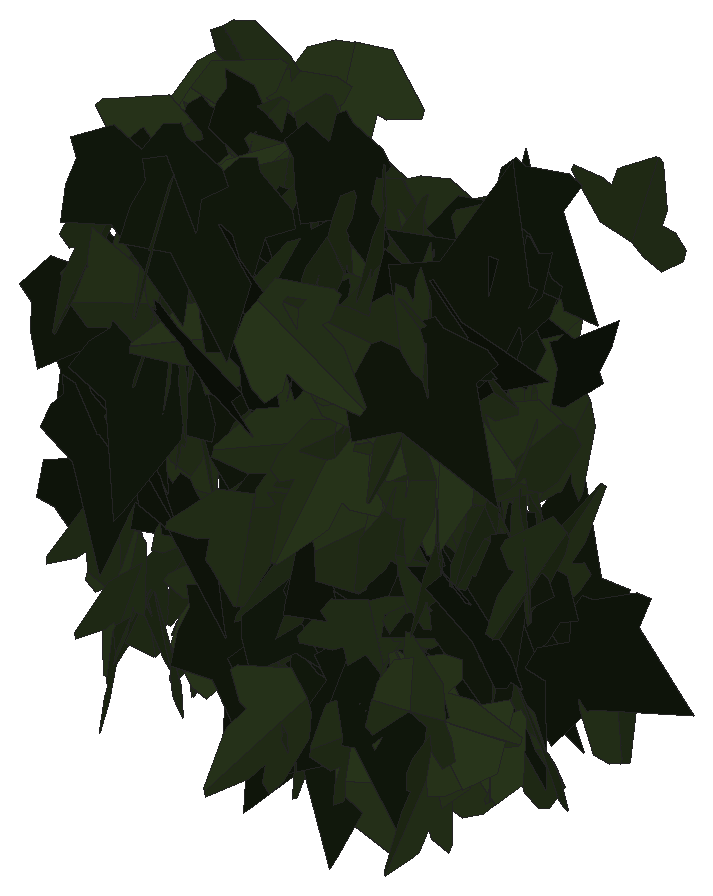
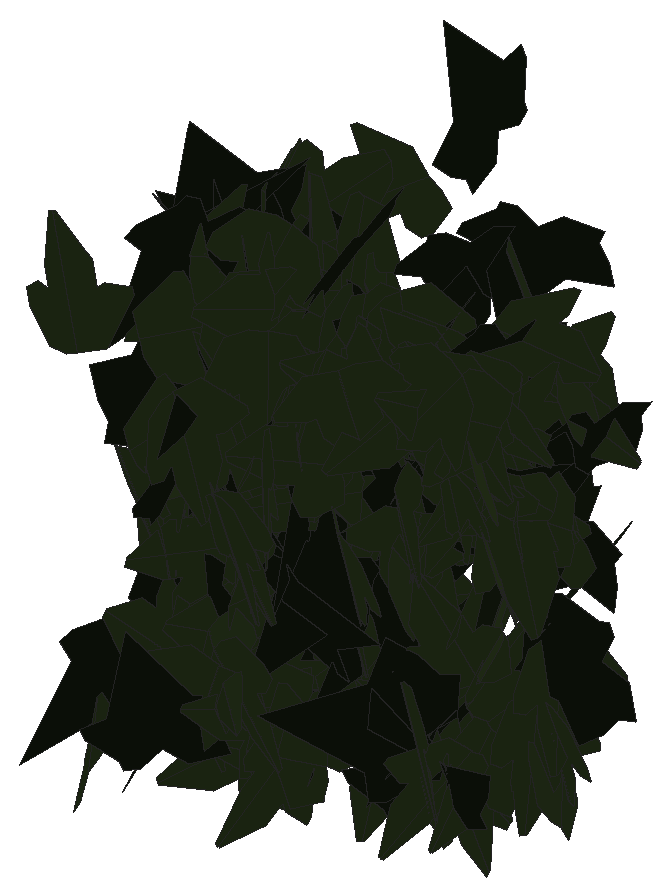
# SketchUp Ruby script. Lengths in inches.
U = 1.inch
M = Sketchup.active_model
def pt(a) = Geom::Point3d.new(a.map { |v| v * U })
def face(e, loops, mat)
  f = e.add_face(loops[0].map { |a| pt(a) })
  loops[1..].each { |l| e.add_face(l.map { |a| pt(a) }).erase! }
  f.material = f.back_material = mat if mat
  f
end
# faces: each face lists its corners as indices into pts; further lists are holes
def faces(e, pts, list, mat = nil) = list.each { |f| face(e, (f[0].is_a?(Array) ? f : [f]).map { |l| l.map { |i| pts[i] } }, mat) }
# xy, xz, yz: faces in a plane at the given z, y or x. An outline is a flat list of corners, or four numbers for a rectangle; further outlines are holes
def ring(l) = l.size == 4 ? [[l[0], l[1]], [l[2], l[1]], [l[2], l[3]], [l[0], l[3]]] : l.each_slice(2).to_a
def flat(e, list, mat, &to3) = list.each { |f| face(e, (f[0].is_a?(Array) ? f : [f]).map { |l| ring(l).map { |u, v| to3.(u, v) } }, mat) }
def xy(e, z, list, mat = nil) = flat(e, list, mat) { |x, y| [x, y, z] }
def xz(e, y, list, mat = nil) = flat(e, list, mat) { |x, z| [x, y, z] }
def yz(e, x, list, mat = nil) = flat(e, list, mat) { |y, z| [x, y, z] }
def lines(e, pts, list) = list.each { |a, b| e.add_line(pt(pts[a]), pt(pts[b])) }
# prism: a flat outline (further loops are holes) pulled along v
def prism(e, loops, v, mat = nil)
  f = face(e, loops, mat); d = Geom::Vector3d.new(v.map { |x| x * U })
  f.pushpull(f.normal.samedirection?(d) ? d.length : -d.length)
end
def box(e, o, s, mat = nil) = prism(e, [[o, [o[0] + s[0], o[1], o[2]], [o[0] + s[0], o[1] + s[1], o[2]], [o[0], o[1] + s[1], o[2]]]], [0, 0, s[2]], mat)
def at(x, y, z, deg = 0) = Geom::Transformation.translation(pt([x, y, z])) * Geom::Transformation.rotation(ORIGIN, Z_AXIS, deg.degrees)
def axes(o, x, y, z) = Geom::Transformation.new([*x, 0, *y, 0, *z, 0, *pt(o).to_a, 1])
def part(name) = M.definitions.add(name)
# library, detail: a bought-in or finely detailed component or shape, given as its bounding box
def library(name, o, s) = part(name).tap { |d| box(d.entities, o, s) }
def detail(e, o, s) = box(e.add_group.entities, o, s)
def put(e, d, t, mat = nil) = e.add_instance(d, t).tap { |i| i.material = mat if mat }
def group(e, t, mat = nil) = e.add_group.tap { |g| g.transformation = t; g.material = mat if mat }.entities
root = M.entities
M.materials.add("efeu1").color = [18, 25, 13]
M.materials.add("efeu2").color = [43, 57, 29]
c1 = part("ivyleaf_10")
p = [[0,0.5,-0.03],[-0.0625,2.02,-0.43],[-0.19,2.01,-0.46],[-0.54,1.05,-0.29],[-0.52,0.625,-0.18],[-0.83,0.76,-0.28],
  [-1.16,0.64,-0.33],[-1.15,0.33,-0.24],[-0.77,-0.39,0.02],[-0.3,-0.51,0.16],[0.04,-0.48,0.23],[-0.02,2.01,-0.4375],
  [-0.06,2.01,-0.43],[0.04,-0.49,0.23],[0.67,-0.49,0.14],[1.38,0.36,-0.2],[1.375,0.51,-0.24],[0.81,0.65,-0.19],
  [0.62,0.59,-0.15],[0.6,1.09,-0.28],[0.5,1.23,-0.31]]
faces(c1.entities,p,[[0,1,2,3,4,5,6,7,8,9,10],[11,12,0,13,14,15,16,17,18,19,20]],"efeu2")
c2 = part("ivyleaf_9")
p = [[1.54,2.16,1.25],[1.36,2.04,1.19],[-0.21,0.99,0.68],[-0.71,1.11,0.82],[-0.85,0.86,0.67],[-0.8,0.17,0.21],
  [-0.9,-0.01,0.1],[-0.67,-0.16,-0.02],[-0.08,-0.08,-0.05],[-0.03,-0.6,-0.4],[0.65,-0.88,-0.66],[0.83,-0.6,-0.49],
  [1.29,-0.42,-0.43],[1.8125,-0.07,-0.26],[1.21,0.44,0.15]]
faces(c2.entities,p,[[0,1,2,3,4,5,6,7,8,9,10,11,12,13,14]],"efeu1")
put(root,c1,axes([18.82,224.73,205.05],[-0.16248,-0.46888,0.06128],[-0.01564,-0.05943,-0.49621],[0.47261,-0.16316,0.00464]))
put(root,c2,axes([18.35,224.16,203.63],[0.15209,-0.02116,-0.47584],[0.38043,0.30596,0.10799],[0.2866,-0.39489,0.10917]))
put(root,c1,axes([18.85,224.05,203.39],[-0.14205,-0.47269,-0.07992],[0.03359,0.07334,-0.49345],[0.47822,-0.14556,0.01092]))
put(root,c1,axes([18.98,224.99,205.75],[0.21391,0.26223,-0.36807],[-0.25951,-0.26212,-0.33756],[-0.36999,0.33546,0.02396]))
put(root,c2,axes([18.71,223.78,205.74],[0.1058,-0.35908,-0.33146],[-0.05142,0.32908,-0.37291],[0.48596,0.113,0.03271]))
put(root,c1,axes([19.1875,224.91,206.44],[0.20931,-0.06031,-0.45006],[-0.43284,0.1233,-0.21782],[0.13726,0.48079,-0.00059]))
put(root,c1,axes([18.84,224.71,206.0625],[0.00108,-0.21736,0.45028],[0.12615,-0.4356,-0.21057],[0.48382,0.11406,0.0539]))
put(root,c1,axes([18.87,223.82,206.3],[0.12744,-0.37917,0.29999],[0.09843,-0.28339,-0.4],[0.47336,0.16101,0.00241]))
put(root,c1,axes([19.04,224.48,206.84],[-0.15279,-0.22328,0.42048],[-0.08154,-0.42281,-0.25414],[0.46905,-0.14623,0.09279]))
put(root,c1,axes([19.31,223.62,205.76],[-0.14542,-0.0502,0.47574],[-0.45603,-0.13566,-0.15371],[0.14451,-0.47862,-0.00633]))
put(root,c1,axes([18.93,224.99,205.14],[0.27965,-0.40943,0.06452],[0.02725,-0.05951,-0.4957],[0.41358,0.28076,-0.01097]))
put(root,c1,axes([19.27,225.18,206.37],[-0.32377,-0.04527,0.37832],[-0.36502,-0.1055,-0.32501],[0.10925,-0.48664,0.03527]))
put(root,c1,axes([18.87,224.15,202.87],[0.42454,-0.2467,0.09436],[0.07894,-0.05195,-0.49099],[0.25206,0.43179,-0.00516]))
put(root,c1,axes([18.99,224.87,203.875],[-0.27867,0.39492,0.12797],[0.05581,-0.11709,0.48288],[0.41137,0.28342,0.02118]))
put(root,c1,axes([18.78,225.84,207.02],[-0.38634,0.14434,-0.28268],[0.26111,-0.10864,-0.41233],[-0.18045,-0.46622,0.00857]))
put(root,c2,axes([18.76,224.01,204.1],[0.04932,-0.44722,0.21809],[0.04765,-0.21391,-0.44941],[0.49527,0.06511,0.02152]))
put(root,c1,axes([18.84,225.22,206.08],[0.22637,-0.30385,0.32624],[0.19886,-0.25865,-0.37889],[0.39901,0.30129,0.00375]))
put(root,c1,axes([18.77,225.36,206.46],[0.13919,0.13008,-0.46228],[0.34562,0.30704,0.19046],[0.33342,-0.37257,-0.00444]))
put(root,c1,axes([19.05,224.13,202.76],[-0.1307,-0.46123,-0.14206],[0.03174,0.13864,-0.47934],[0.48157,-0.13432,-0.00696]))
put(root,c1,axes([18.9,224.05,201.97],[0.06033,-0.33427,-0.36691],[0.10611,-0.35238,0.33848],[-0.48487,-0.11871,0.02842]))
put(root,c2,axes([18.82,223.99,204.8125],[-0.20178,-0.10215,-0.44593],[0.3856,0.22428,-0.22585],[0.24616,-0.43505,-0.01173]))
put(root,c1,axes([18.88,224.49,205.09],[0.00643,-0.04596,0.49784],[0.28534,-0.4085,-0.04139],[0.41054,0.28464,0.02098]))
put(root,c2,axes([18.93,224.42,205.11],[-0.10806,-0.06374,0.484],[0.40936,0.25825,0.12541],[-0.26598,0.42337,-0.00363]))
put(root,c1,axes([19.08,224.32,205.4],[0.01022,-0.09092,-0.49156],[0.05311,0.48908,-0.08935],[0.49707,-0.05038,0.01966]))
put(root,c1,axes([18.69,224.38,205.05],[0.00757,-0.03332,0.49883],[0.4858,0.1183,0.00053],[-0.11806,0.48466,0.03416]))
put(root,c1,axes([19.09,224.88,202.74],[-0.04363,-0.31774,-0.38358],[0.07395,0.37665,-0.32041],[0.49257,-0.08469,0.01413]))
put(root,c1,axes([18.73,224.14,204.83],[0.21599,0.00441,0.45092],[0.44977,0.03395,-0.21577],[-0.03252,0.49883,0.0107]))
put(root,c2,axes([19.14,224.88,205.32],[-0.25843,-0.39915,0.15459],[-0.06902,-0.13935,-0.4752],[0.42244,-0.26695,0.01692]))
put(root,c1,axes([19.125,224.75,203.36],[-0.12305,0.28413,0.39259],[0.09482,-0.38311,0.30698],[0.47526,0.15,0.0404]))
put(root,c1,axes([19.26,225.66,203.48],[0.25427,-0.35532,-0.24309],[-0.1462,0.19428,-0.4369],[0.40494,0.29326,-0.0051]))
put(root,c1,axes([18.9,225.32,206.73],[0.17967,0.21339,0.41495],[0.27566,0.31021,-0.27889],[-0.37647,0.32898,-0.00617]))
put(root,c1,axes([19.02,225.2,206.18],[-0.30688,-0.30797,0.24694],[0.18765,0.16137,0.43445],[-0.3473,0.35932,0.01653]))
put(root,c1,axes([18.97,224.89,205.41],[0.25172,0.32401,0.28575],[0.18023,0.2218,-0.41027],[-0.39263,0.30955,-0.00513]))
put(root,c2,axes([18.87,223.97,204.59],[0.26386,-0.36724,0.21334],[0.11545,-0.17968,-0.45209],[0.40871,0.28784,-0.01003]))
put(root,c1,axes([19.07,225.35,202.79],[0.07555,0.37256,0.32479],[0.07553,0.316,-0.38005],[-0.48845,0.10649,-0.00853]))
put(root,c1,axes([19.44,225.55,205.45],[0.09881,-0.09151,-0.48152],[-0.26261,0.40487,-0.13083],[0.41385,0.27876,0.03194]))
put(root,c1,axes([19.36,223.97,205.02],[0.30601,-0.30238,-0.25479],[-0.15928,0.20062,-0.42939],[0.36192,0.34397,0.02646]))
put(root,c2,axes([19.11,224.55,206.8],[0.03533,-0.33452,-0.36993],[-0.05415,0.36609,-0.33622],[0.4958,0.06383,-0.01036]))
put(root,c1,axes([19.17,224.8,204.49],[-0.15727,0.45329,-0.1407],[0.04663,-0.13275,-0.4798],[-0.47233,-0.16403,-0.00052]))
put(root,c1,axes([19.08,225.125,203.78],[0.43431,0.12721,-0.21258],[0.20414,0.0593,0.45256],[0.14035,-0.4799,-0.00043]))
put(root,c1,axes([19.19,225.22,205.6875],[0.43726,-0.21905,0.10404],[0.09234,-0.04796,-0.48905],[0.22423,0.4469,-0.00149]))
put(root,c1,axes([19.3,224.6,205.46],[-0.00131,-0.17139,-0.46971],[0.08985,0.46198,-0.16882],[0.49186,-0.08485,0.02959]))
put(root,c1,axes([19.37,224.91,202.41],[0.06659,-0.48362,0.10804],[0.00692,-0.10809,-0.48813],[0.4955,0.0665,-0.00771]))
put(root,c1,axes([19.4,224.25,204.66],[-0.25469,-0.37816,-0.20525],[-0.08649,-0.18865,0.4549],[-0.42149,0.26722,0.03068]))
put(root,c1,axes([19.48,224.92,206.14],[-0.09905,-0.3584,0.33427],[-0.03897,-0.33419,-0.36986],[0.48854,-0.09932,0.03827]))
put(root,c1,axes([19.47,224.875,202.58],[-0.07117,-0.39536,0.2977],[-0.02394,-0.29766,-0.40103],[0.49433,-0.07134,0.02344]))
put(root,c1,axes([19.29,224.04,205.16],[0.11397,-0.46404,-0.14724],[0.04644,-0.14017,0.4777],[-0.48462,-0.12256,0.01115]))
put(root,c1,axes([19.23,225.7,206.65],[-0.29503,-0.17441,-0.36406],[0.32053,0.1729,-0.34259],[0.24539,-0.43553,0.00979]))
put(root,c2,axes([19.38,225.4,202.36],[-0.39083,0.04109,0.30914],[0.3026,-0.06987,0.39185],[0.0754,0.49339,0.02974]))
put(root,c1,axes([19.36,225.14,206.48],[0.30739,-0.33161,0.21341],[0.14181,-0.15953,-0.45215],[0.36797,0.3385,-0.00403]))
put(root,c1,axes([19.56,225.125,203.13],[0.36656,-0.3399,-0.01009],[-0.00849,0.00568,-0.4999],[0.33995,0.36665,-0.00161]))
put(root,c2,axes([19.4,225.39,202.9],[0.02857,-0.48837,0.10334],[0.01144,-0.10284,-0.48918],[0.49905,0.03031,0.0053]))
put(root,c2,axes([19.49,223.84,205.09],[-0.11325,-0.47305,0.11573],[-0.01642,-0.11505,-0.48631],[0.48673,-0.11395,0.01052]))
put(root,c1,axes([19.49,224.48,205.73],[0.23719,-0.34544,0.27278],[0.19011,-0.19908,-0.41741],[0.39699,0.30173,0.0369]))
put(root,c1,axes([19.61,223.82,202.22],[-0.39451,0.26975,0.14698],[0.11682,-0.08952,0.47785],[0.28411,0.41137,0.0076]))
put(root,c1,axes([19.61,226.21,206.92],[0.35284,0.33763,-0.10728],[-0.07664,-0.07509,-0.48835],[-0.34588,0.36106,-0.00124]))
put(root,c1,axes([19.36,225.44,202.84],[0.1431,-0.14805,0.45564],[0.38754,-0.2438,-0.20093],[0.28166,0.41066,0.04497]))
put(root,c2,axes([19.3,225.51,203.16],[0.24406,0.04256,0.43431],[0.42628,0.08323,-0.24771],[-0.09338,0.49118,0.00434]))
put(root,c2,axes([19.49,225.29,206.79],[0.09012,-0.45959,0.1751],[0.03098,-0.17235,-0.46833],[0.49084,0.09526,-0.00259]))
put(root,c1,axes([19.47,224.37,206.24],[0.31185,0.12323,-0.3709],[0.33661,0.15643,0.335],[0.1986,-0.45863,0.01461]))
put(root,c2,axes([19.6,223.46,207.32],[-0.21592,-0.28961,-0.34569],[0.20925,0.27517,-0.36124],[0.39949,-0.30067,0.00237]))
put(root,c1,axes([19.44,225.15,202.74],[-0.20531,-0.02359,0.45529],[0.45066,0.06501,0.20659],[-0.06895,0.49519,-0.00544]))
put(root,c1,axes([19.73,223.54,206.89],[0.31268,-0.36305,0.14293],[0.09031,-0.11085,-0.47912],[0.37957,0.32544,-0.00375]))
put(root,c2,axes([19.52,223.99,203.85],[0.2185,-0.42301,0.15272],[0.08076,-0.13013,-0.47597],[0.44242,0.23266,0.01146]))
put(root,c1,axes([19.66,224.59,205.57],[-0.24056,0.13641,0.41656],[0.3303,-0.25596,0.27457],[0.28815,0.40728,0.03303]))
put(root,c1,axes([19.64,223.94,204.89],[-0.0568,0.02356,0.4962],[0.3945,-0.30138,0.05947],[0.30189,0.39827,0.01565]))
put(root,c1,axes([19.75,224.87,202.38],[-0.39283,-0.04192,0.30647],[0.305,0.03009,0.39506],[-0.05157,0.49733,0.00193]))
put(root,c1,axes([19.96,224.83,204.36],[0.10926,-0.40453,0.2728],[0.05081,-0.2686,-0.41865],[0.48526,0.1192,-0.01758]))
put(root,c1,axes([19.65,224.8,206.53],[0.28898,0.12113,0.38964],[0.36012,0.14878,-0.31334],[-0.19185,0.46173,-0.00125]))
put(root,c1,axes([20.22,224.12,205.56],[-0.02686,0.04078,0.49761],[-0.2124,-0.45192,0.02558],[0.45184,-0.21001,0.0416]))
put(root,c2,axes([19.8125,224.46,205.74],[0.24428,-0.41888,-0.12193],[-0.0616,0.10522,-0.48491],[0.43189,0.25193,-0.0002]))
put(root,c1,axes([19.93,224.73,204.68],[0.38998,0.30569,0.06686],[0.05063,0.04378,-0.4955],[-0.30879,0.39324,0.00319]))
put(root,c1,axes([20.12,224.7,206.76],[-0.1385,-0.4804,0.00614],[-0.00172,-0.0059,-0.49996],[0.48043,-0.13851,-0.00002]))
put(root,c1,axes([19.95,225.74,204.92],[0.39828,-0.26334,0.14841],[0.1236,-0.08215,-0.47747],[0.27586,0.41702,-0.00034]))
put(root,c2,axes([20.1,224.39,202.74],[-0.35522,0.04508,-0.34898],[0.34589,-0.04637,-0.35806],[-0.06465,-0.4958,0.00176]))
put(root,c1,axes([19.78,225.64,206.4375],[-0.04279,-0.03643,0.49683],[0.48794,0.09745,0.04917],[-0.10041,0.48906,0.02721]))
put(root,c1,axes([19.94,224.02,202.72],[0.18389,0.26122,0.38464],[0.19062,0.33492,-0.31858],[-0.42409,0.26381,0.0236]))
put(root,c1,axes([19.88,225.34,203.64],[0.30852,-0.09705,0.38131],[0.36105,-0.12276,-0.32337],[0.15639,0.47488,-0.00567]))
put(root,c1,axes([19.875,224.94,202.8],[0.12523,-0.09843,-0.47395],[0.41347,0.27632,0.05187],[0.25171,-0.40492,0.15061]))
put(root,c1,axes([20.25,224.3125,204.38],[0.17264,-0.42808,-0.19221],[-0.02469,0.19624,-0.45922],[0.4686,0.16805,0.04662]))
put(root,c2,axes([19.9375,224.77,206.26],[0.27999,-0.4045,0.08937],[0.05368,-0.07153,-0.49194],[0.41076,0.28507,0.00337]))
put(root,c2,axes([20.14,223.73,207.09],[-0.16949,-0.41564,-0.22026],[0.08883,0.20163,-0.44884],[0.46193,-0.19128,0.00549]))
put(root,c2,axes([20.29,224.47,203.875],[0.03999,-0.03093,-0.49744],[-0.22059,0.4464,-0.04549],[0.44692,0.2231,0.02206]))
put(root,c2,axes([20,224.375,204.81],[0.04455,-0.13735,-0.4787],[0.32669,0.37081,-0.07599],[0.37588,-0.306,0.12278]))
put(root,c2,axes([20.05,224.76,206.36],[0.03096,-0.01223,-0.49889],[0.2173,0.45031,0.00245],[0.44925,-0.21697,0.0332]))
put(root,c1,axes([20.39,224.88,206.67],[0.01507,-0.48313,0.12791],[0.00736,-0.12774,-0.48335],[0.49972,0.01645,0.00326]))
put(root,c2,axes([20.19,224.09,202.79],[0.03569,-0.49494,-0.06134],[-0.00497,0.06114,-0.49622],[0.4987,0.03603,-0.00056]))
put(root,c1,axes([20.14,224.6,204.66],[-0.2258,0.2314,-0.3814],[0.27713,-0.26222,-0.32317],[-0.34959,-0.35734,-0.00984]))
put(root,c2,axes([20,223.89,206.28],[0.17289,0.01979,-0.46874],[0.45884,0.09707,0.17333],[0.09786,-0.49009,0.0154]))
put(root,c1,axes([20.71,224.95,206.34],[-0.217,0.15992,-0.42111],[-0.32918,0.26278,0.26942],[0.30749,0.39417,-0.00876]))
put(root,c2,axes([20.82,225.52,203.98],[-0.34216,-0.02313,-0.36385],[-0.3567,-0.082,0.34065],[-0.07543,0.49269,0.03961]))
put(root,c1,axes([20.47,224.59,206.18],[-0.04001,-0.49561,0.05264],[-0.00197,-0.05265,-0.49722],[0.49839,-0.04,0.00226]))
put(root,c1,axes([20.35,224.89,202.91],[-0.02966,-0.49774,-0.0371],[0.0127,-0.0379,0.4984],[-0.49896,0.02862,0.01489]))
put(root,c1,axes([20.4,225.29,206.7],[-0.00413,0.3929,-0.30921],[-0.03358,-0.30874,-0.39185],[-0.49885,0.01753,0.02894]))
put(root,c1,axes([20.47,224.51,202.33],[-0.26006,-0.40367,-0.13935],[0.08046,0.11392,-0.48015],[0.4194,-0.27216,0.0057]))
put(root,c1,axes([20.66,224.95,204.17],[0.29158,-0.34881,-0.20811],[-0.13382,0.15939,-0.45463],[0.3835,0.32082,-0.00041]))
put(root,c1,axes([20.24,225.78,205.73],[0.1024,-0.03732,0.48798],[0.46969,0.14756,-0.08728],[-0.13749,0.47627,0.06528]))
put(root,c2,axes([20.46,225.23,204.39],[0.48861,0.08248,-0.06676],[-0.06583,-0.0111,-0.49552],[-0.08323,0.49302,0.00001]))
put(root,c2,axes([20.63,224.4,206.5],[-0.42246,-0.06925,-0.25833],[0.25403,0.04716,-0.42807],[0.08365,-0.49293,-0.00467]))
put(root,c1,axes([20.78,225.86,205.5625],[0.18046,-0.26598,-0.383],[-0.14558,0.35801,-0.31722],[0.44299,0.22601,0.05177]))
put(root,c1,axes([20.85,226.32,205.18],[0.37298,-0.1899,-0.27354],[-0.23027,0.1496,-0.41784],[0.24054,0.43767,0.02414]))
put(root,c2,axes([20.85,225.13,205.14],[0.07937,-0.0399,-0.49204],[-0.40326,0.28222,-0.08794],[0.28475,0.4108,0.01262]))
put(root,c1,axes([20.8,224.67,204.9],[-0.16921,-0.46999,-0.02184],[0.00711,0.02066,-0.49952],[0.47044,-0.16936,-0.00031]))
put(root,c1,axes([20.53,224.72,205.51],[-0.29456,-0.19349,0.35468],[0.29637,0.19484,0.35242],[-0.27459,0.41785,-0.00009]))
put(root,c1,axes([20.82,224.97,205.68],[-0.4771,-0.14957,0.00295],[-0.00235,-0.00237,-0.49999],[0.14958,-0.4771,0.00156]))
put(root,c2,axes([20.4375,223.76,205.45],[0.0496,-0.0657,0.49318],[0.30443,-0.38801,-0.08231],[0.39353,0.30844,0.00151]))
put(root,c1,axes([20.84,223.99,203.57],[-0.00126,-0.49982,-0.01343],[-0.00062,0.01343,-0.49982],[0.5,-0.00124,-0.00065]))
put(root,c1,axes([20.65,224.6,205.48],[0.11971,0.32442,0.36114],[0.11173,0.34356,-0.34566],[-0.47243,0.16346,0.00976]))
put(root,c1,axes([20.55,225.65,205.92],[-0.12286,0.07338,0.47908],[0.40308,-0.25897,0.14303],[0.26913,0.42137,0.00448]))
put(root,c1,axes([20.87,226.32,205.17],[0.38189,-0.30821,-0.09577],[-0.07555,0.05887,-0.49074],[0.31378,0.38928,-0.00161]))
put(root,c2,axes([21.02,224.75,204.7],[-0.30166,-0.27049,0.29298],[-0.22173,-0.19155,-0.40515],[0.33141,-0.37436,-0.00438]))
put(root,c1,axes([21.06,224.1,202.18],[0.34309,-0.10161,0.34924],[-0.33424,0.10126,0.35781],[-0.14344,-0.47898,0.00156]))
put(root,c1,axes([21.12,225.93,203.33],[0.27274,-0.16745,-0.38415],[-0.31181,0.22512,-0.31952],[0.27997,0.41386,0.01838]))
put(root,c1,axes([21,225.14,202.63],[-0.13244,-0.27689,0.39471],[-0.05934,-0.39685,-0.2983],[0.47847,-0.12586,0.07226]))
put(root,c1,axes([20.85,225.49,202.35],[-0.04458,-0.28484,-0.40851],[0.15075,0.38318,-0.28363],[0.47464,-0.14846,0.05172]))
put(root,c1,axes([20.9,224.72,203.46],[-0.04434,-0.16147,0.47113],[0.10022,-0.46621,-0.15036],[0.48784,0.0811,0.07371]))
put(root,c1,axes([20.95,224.48,205.11],[-0.10789,-0.3575,0.33249],[0.04203,-0.34605,-0.35844],[0.48641,-0.0494,0.10473]))
put(root,c2,axes([20.75,224.4375,202.93],[-0.13451,0.29147,0.38334],[0.1629,-0.34701,0.32101],[0.45318,0.21125,-0.00161]))
put(root,c2,axes([20.82,223.98,202.3],[-0.03316,-0.38519,0.31706],[-0.02569,-0.31602,-0.38661],[0.49824,-0.04193,0.00117]))
put(root,c2,axes([20.76,224.57,207.3125],[0.23619,-0.41305,-0.15362],[-0.06868,0.13767,-0.47574],[0.43531,0.24583,0.00829]))
put(root,c1,axes([21.09,223.07,204.58],[-0.34231,-0.35848,0.06569],[-0.04072,-0.05194,-0.49563],[0.36217,-0.34466,0.00636]))
put(root,c1,axes([21.27,224.05,204.48],[0.06699,-0.02952,-0.49461],[-0.34841,0.35208,-0.0682],[0.35231,0.35379,0.0266]))
put(root,c1,axes([21.22,225.34,202.83],[-0.00083,-0.02421,0.49941],[-0.24819,-0.43352,-0.02143],[0.43405,-0.24793,-0.01129]))
put(root,c1,axes([20.66,225.5,202.4],[0.01058,-0.02557,0.49923],[0.44866,0.22068,0.00179],[-0.22043,0.44794,0.02762]))
put(root,c2,axes([20.89,224.34,203.42],[0.36031,0.31541,0.14385],[0.10666,0.09656,-0.47885],[-0.32985,0.37576,0.0023]))
put(root,c1,axes([20.76,224.91,204.79],[0.10607,-0.09166,-0.47995],[0.37893,0.32549,0.02158],[0.30848,-0.36831,0.13851]))
put(root,c2,axes([20.9,225.18,202.09],[-0.09133,0.0017,0.49158],[0.04836,-0.49754,0.0107],[0.4892,0.0495,0.09072]))
put(root,c1,axes([21.05,224.01,203.28],[-0.10125,-0.4103,-0.26721],[0.07285,0.2572,-0.42254],[0.48419,-0.1245,0.0077]))
put(root,c1,axes([21.32,223.87,203.04],[0.14798,-0.12208,-0.46173],[-0.34659,0.30513,-0.19176],[0.3286,0.37682,0.00568]))
put(root,c2,axes([20.89,223.92,203.53],[0.0877,-0.33417,-0.36144],[0.00116,0.36727,-0.33928],[0.49225,0.05867,0.0652]))
put(root,c1,axes([21.33,224.86,206.06],[-0.21864,-0.257,0.36898],[-0.2166,-0.29936,-0.33685],[0.39406,-0.30714,0.01957]))
put(root,c1,axes([21.24,225.33,206.23],[-0.48521,-0.08471,0.08602],[-0.08376,-0.02037,-0.49251],[0.08695,-0.49235,0.00557]))
put(root,c1,axes([21.17,225.1,205.53],[0.06615,-0.10335,-0.48471],[-0.00773,0.48873,-0.10526],[0.49554,0.02142,0.06307]))
put(root,c1,axes([21.45,224.34,203.47],[-0.00296,0.01702,0.4997],[-0.3786,-0.32647,0.00887],[0.32658,-0.37832,0.01482]))
put(root,c1,axes([21.04,223.94,206.3125],[0.30345,-0.33126,0.21951],[0.13475,-0.17405,-0.44894],[0.37384,0.33162,-0.01635]))
put(root,c1,axes([21.33,224.49,202.36],[0.14681,-0.2662,-0.39696],[-0.19329,0.34673,-0.304],[0.43713,0.24272,-0.0011]))
put(root,c1,axes([21.2,225.11,204.7],[-0.14272,-0.43188,-0.20763],[0.05695,0.19982,-0.45478],[0.4758,-0.15347,-0.00785]))
put(root,c1,axes([21.42,225.73,203.36],[0.21357,-0.00373,-0.45208],[-0.27512,0.39568,-0.13324],[0.35875,0.30566,0.16695]))
put(root,c1,axes([21.04,223.77,202.18],[-0.21457,0.14394,0.42807],[0.29482,-0.31437,0.25349],[0.34212,0.36118,0.05003]))
put(root,c1,axes([21,225.36,202.74],[0.10461,0.05868,-0.4854],[0.30687,0.37856,0.1119],[0.38064,-0.32132,0.04318]))
put(root,c1,axes([21.07,224.375,203.4],[0.02733,-0.12659,-0.48294],[0.25682,0.41833,-0.09512],[0.42813,-0.24285,0.08788]))
put(root,c1,axes([21.27,225.15,206.1],[-0.49948,-0.01898,-0.01271],[0.01272,-0.00001,-0.49984],[0.01897,-0.49964,0.00049]))
put(root,c1,axes([21.32,223.8,206.93],[0.02514,-0.39194,-0.30943],[-0.01859,0.30888,-0.39275],[0.49902,0.03125,0.00096]))
put(root,c1,axes([21.3,223.48,205.16],[-0.04378,0.16561,0.46974],[0.02183,-0.47046,0.1679],[0.4976,0.03521,0.03397]))
put(root,c2,axes([21.11,224.17,203.64],[0.26155,-0.24954,-0.34543],[0.25229,-0.23597,0.36149],[-0.34343,-0.36339,0.00248]))
put(root,c1,axes([21.45,224.37,206.14],[-0.44251,-0.20483,0.11059],[-0.1002,-0.04679,-0.48762],[0.2101,-0.45371,0.00036]))
put(root,c1,axes([21.39,226.3125,206],[-0.06541,-0.49158,0.06383],[-0.0036,-0.06391,-0.49589],[0.49569,-0.06533,0.00482]))
put(root,c2,axes([21.07,224.14,205.5],[-0.12208,-0.16464,-0.45606],[0.35264,0.29263,-0.20003],[0.33278,-0.37049,0.04467]))
put(root,c1,axes([21.43,223.84,205.75],[0.46794,-0.06656,-0.1631],[-0.16178,0.02082,-0.47265],[0.06971,0.49511,-0.00205]))
put(root,c1,axes([21.32,225.43,203.77],[-0.07277,-0.05304,0.49182],[0.14964,-0.47619,-0.02921],[0.4715,0.14294,0.08518]))
put(root,c1,axes([21.39,223.11,202.7],[-0.09618,-0.12613,0.47417],[0.07743,-0.48104,-0.11226],[0.48451,0.05184,0.11207]))
put(root,c1,axes([21.44,225.54,205.64],[0.07422,-0.48716,0.08466],[0.00452,-0.08493,-0.49271],[0.49444,0.07391,-0.00821]))
put(root,c1,axes([21.46,223.7,205.04],[-0.1277,-0.4738,-0.09596],[0.01442,0.09547,-0.49059],[0.4832,-0.12806,-0.01072]))
put(root,c1,axes([21.48,224.7,204.02],[-0.16792,-0.46319,-0.08519],[0.02611,0.08114,-0.49268],[0.47023,-0.16991,-0.00306]))
put(root,c1,axes([21.45,224.04,205.99],[0.02079,0.05485,0.49655],[-0.06192,0.49343,-0.05191],[-0.49572,-0.05933,0.02731]))
put(root,c1,axes([21.27,225.98,203.21],[0.44821,0.11208,0.19118],[0.18211,0.05952,-0.46184],[-0.12628,0.48363,0.01253]))
put(root,c2,axes([21.19,224.27,204.28],[0.14772,0.32714,-0.34808],[0.13999,0.3187,0.35893],[0.45671,-0.2035,0.00256]))
put(root,c1,axes([21.51,223.62,205.04],[0.16571,0.3551,-0.31055],[-0.12446,-0.28458,-0.39182],[-0.45503,0.20716,-0.00592]))
put(root,c1,axes([21.8,225,206.35],[-0.15851,-0.15189,0.44923],[-0.33821,-0.2958,-0.21935],[0.3324,-0.3734,-0.00896]))
put(root,c2,axes([21.59,226.15,205.23],[-0.12956,-0.29741,0.38048],[0.15084,0.3493,0.3244],[-0.45876,0.19884,-0.00078]))
put(root,c2,axes([21.48,223.95,202.56],[-0.28836,-0.37054,-0.1719],[0.10545,0.13575,-0.46952],[0.39463,-0.30704,-0.00014]))
put(root,c1,axes([21.63,223.81,202.53],[-0.43232,0.23362,0.09232],[-0.08142,0.04351,-0.4914],[-0.23764,-0.43992,0.00042]))
put(root,c1,axes([21.64,224.1,207.18],[0.17839,-0.37915,-0.27281],[-0.07189,0.26626,-0.41706],[0.46153,0.18802,0.04048]))
put(root,c1,axes([21.625,224.81,203.99],[-0.07922,-0.44038,-0.22314],[0.01993,0.22296,-0.44709],[0.49328,-0.07974,-0.01777]))
put(root,c1,axes([21.52,224.75,206.41],[0.0198,-0.18129,0.46556],[0.00581,0.46597,0.1812],[-0.49957,-0.00177,0.02056]))
put(root,c1,axes([21.72,224.41,204.24],[-0.42885,-0.23799,0.0972],[-0.07874,-0.05835,-0.4903],[0.24472,-0.43584,0.01257]))
put(root,c2,axes([21.25,223.91,203.56],[0.06291,-0.04682,-0.49381],[0.30337,0.39745,0.00097],[0.39244,-0.29974,0.07841]))
put(root,c1,axes([21.56,224.75,207.02],[-0.47155,-0.0342,-0.1627],[0.16309,-0.00015,-0.47265],[0.03229,-0.49883,0.0113]))
put(root,c1,axes([21.55,223.9,202.27],[-0.14321,0.13653,0.45918],[0.21865,-0.4078,0.18945],[0.42624,0.25506,0.05709]))
put(root,c1,axes([21.82,224.85,203.78],[-0.01419,0.19699,-0.45934],[-0.15457,0.43527,0.19144],[0.4753,0.14743,0.04855]))
put(root,c2,axes([21.74,223.95,205.99],[0.26876,0.3651,-0.21087],[-0.13131,-0.16515,-0.4533],[-0.40065,0.29904,0.00711]))
put(root,c2,axes([21.66,224.67,205.6],[0.3799,0.09449,0.31105],[-0.30224,-0.07351,0.39147],[0.11971,-0.48546,0.00127]))
put(root,c2,axes([21.9,224.03,202.76],[0.00951,0.02212,-0.49942],[-0.12098,-0.48456,-0.02376],[-0.48505,0.1213,-0.00387]))
put(root,c1,axes([21.55,223.64,204.27],[0.01505,0.04505,-0.49774],[0.24901,0.43108,0.04654],[0.43332,-0.24929,-0.00946]))
put(root,c2,axes([21.69,225.15,204.48],[-0.40931,-0.04932,-0.2829],[0.27933,0.04596,-0.41215],[0.06666,-0.49543,-0.01007]))
put(root,c1,axes([21.57,224.99,202.11],[-0.08225,-0.1075,-0.48133],[0.29944,0.37685,-0.13534],[0.39188,-0.31052,0.00239]))
put(root,c1,axes([21.74,224.64,204.51],[-0.09424,-0.19146,0.45217],[0.09979,-0.45829,-0.17325],[0.48079,0.05759,0.12459]))
put(root,c2,axes([21.77,226.13,202.45],[-0.34853,-0.13433,0.33238],[0.33226,0.05308,0.36985],[-0.13465,0.47868,0.05226]))
put(root,c1,axes([21.84,224.55,202.8],[0.44498,-0.16965,0.15235],[-0.13898,0.06306,0.47614],[-0.18077,-0.46609,0.00896]))
put(root,c1,axes([21.77,224.97,203.03],[0.03883,-0.2572,0.42701],[-0.02247,0.42697,0.25922],[-0.49798,-0.03932,0.0216]))
put(root,c1,axes([21.86,223.77,203.52],[-0.41974,-0.26595,-0.05561],[0.05215,0.02158,-0.4968],[0.26665,-0.42285,0.00962]))
put(root,c1,axes([21.57,224.56,204.64],[-0.2176,0.06147,0.44595],[0.43066,-0.11578,0.2261],[0.13106,0.48251,-0.00255]))
put(root,c1,axes([21.85,224.5625,202.59],[0.3421,-0.3624,0.04045],[0.03199,-0.02543,-0.49833],[0.36324,0.34354,0.00578]))
put(root,c1,axes([21.7,224.74,204.12],[-0.36809,-0.17061,0.29224],[0.2645,0.12427,0.4057],[-0.21107,0.45327,-0.00123]))
put(root,c2,axes([21.52,221.65,206.92],[0.38084,-0.04574,-0.32073],[0.31907,-0.03284,0.38356],[-0.05616,-0.49682,0.00418]))
put(root,c1,axes([21.5625,223.49,205.9],[-0.15488,-0.09258,0.4663],[0.43166,0.17811,0.17874],[-0.1992,0.45794,0.02476]))
put(root,c1,axes([21.77,225.2,202.25],[-0.0198,0.01685,0.49932],[0.24323,-0.43617,0.02436],[0.4364,0.24386,0.00907]))
put(root,c2,axes([21.61,224.63,202.65],[0.11098,0.04848,0.48511],[0.46632,0.13459,-0.12014],[-0.14223,0.4791,-0.01534]))
put(root,c1,axes([21.92,224.98,204.08],[-0.18659,-0.34904,-0.30555],[0.12961,0.277,-0.39557],[0.44541,-0.22682,-0.01289]))
put(root,c2,axes([22.33,225.3,203.57],[-0.04988,-0.03743,-0.4961],[-0.40425,-0.28757,0.06234],[-0.28999,0.40731,-0.00158]))
put(root,c2,axes([22.16,224.14,202.48],[0.22869,0.00723,0.44458],[-0.44061,0.07083,0.22549],[-0.05972,-0.4949,0.03877]))
put(root,c1,axes([21.9,225.18,204.02],[0.02521,-0.12339,0.48388],[0.01927,0.48438,0.12251],[-0.49899,0.01248,0.02918]))
put(root,c1,axes([21.66,222.6875,206.76],[0.24743,0.11675,0.41851],[0.38519,0.16387,-0.27345],[-0.20101,0.45773,-0.00885]))
put(root,c2,axes([21.85,224.1875,204.07],[0.48036,-0.04053,-0.13272],[-0.13213,0.01251,-0.48206],[0.04239,0.4982,0.00131]))
put(root,c1,axes([22.11,225.77,205.32],[0.0163,0.19605,0.45967],[-0.04797,-0.45718,0.19669],[0.49743,-0.05051,0.00391]))
put(root,c2,axes([21.89,224.68,205.42],[-0.06651,0.37494,0.32403],[0.05036,-0.32013,0.38077],[0.49299,0.08329,0.00482]))
put(root,c1,axes([21.74,225,202.5],[0.13839,0.14498,0.45807],[0.32873,0.31909,-0.2003],[-0.35041,0.3566,-0.00701]))
put(root,c1,axes([22.08,224.33,203.28],[0.03815,-0.34121,0.36348],[0.02103,-0.36312,-0.34308],[0.4981,0.04146,-0.01335]))
put(root,c1,axes([22.2,224.54,205.16],[-0.02394,0.07471,0.49381],[-0.10506,-0.48407,0.06814],[0.48825,-0.1005,0.03888]))
put(root,c2,axes([21.95,225.41,202.87],[0.29651,-0.30667,-0.26084],[-0.17209,0.19632,-0.42643],[0.36396,0.34266,0.01087]))
put(root,c1,axes([22.35,223.3,206.47],[-0.22533,-0.13791,-0.42451],[-0.35977,-0.22534,0.26418],[-0.26419,0.4245,0.00232]))
put(root,c1,axes([21.97,224.85,204.28],[0.02785,-0.3544,-0.35161],[0.09418,-0.3421,0.35228],[-0.49026,-0.08585,0.04771]))
put(root,c1,axes([22.08,223.77,204.58],[-0.0911,-0.34887,-0.3464],[0.12483,0.32433,-0.35948],[0.47552,-0.15198,0.028]))
put(root,c1,axes([22.11,225.67,203.0625],[0.09258,-0.3641,0.32994],[-0.0571,0.3255,0.37522],[-0.48802,-0.10716,0.01869]))
put(root,c1,axes([22.375,225.21,204.35],[-0.11794,0.23243,-0.42669],[-0.22338,0.36399,0.26002],[0.4315,0.25196,0.01798]))
put(root,c2,axes([21.97,223.71,202.98],[-0.26792,-0.15758,-0.39165],[0.35224,0.17223,-0.31026],[0.23269,-0.44216,0.01872]))
put(root,c1,axes([22.33,223.67,204.31],[-0.14424,0.21755,0.42646],[-0.23924,0.35304,-0.26101],[-0.41468,-0.27935,0.00225]))
put(root,c1,axes([22.43,225.2,206],[0.06717,0.09325,0.48661],[-0.27006,-0.40482,0.11486],[0.4154,-0.27826,-0.00401]))
put(root,c1,axes([22.58,223.63,202.9],[-0.11507,0.02603,0.48588],[-0.48652,0.00197,-0.11532],[-0.00792,-0.49932,0.02488]))
put(root,c1,axes([22.1875,224.43,205.8],[0.12099,-0.43266,0.21946],[0.07693,-0.20621,-0.44895],[0.479,0.14241,0.01667]))
put(root,c1,axes([21.83,223.68,202],[0.09834,-0.06337,-0.48612],[0.48835,-0.03077,0.10281],[-0.04295,-0.49501,0.05584]))
put(root,c1,axes([22.24,223.89,205.8],[0.06045,-0.39267,0.30358],[0.07397,-0.29528,-0.39666],[0.49079,0.09286,0.02239]))
put(root,c1,axes([22.2,224.89,206.75],[0.0468,-0.20115,0.45535],[0.13271,-0.43577,-0.20614],[0.47979,0.14015,0.0126]))
put(root,c1,axes([22.52,223.51,205.21],[0.18986,-0.16128,-0.43352],[-0.33203,0.27875,-0.24911],[0.32204,0.38247,-0.00125]))
put(root,c1,axes([22.35,224.9375,205.74],[0.42096,-0.20684,-0.17323],[-0.14859,0.09021,-0.46881],[0.22519,0.44618,0.01448]))
put(root,c2,axes([22.08,224.61,206.22],[-0.03787,0.13568,0.47975],[0.16166,-0.45179,0.14053],[0.47163,0.16576,-0.00965]))
put(root,c1,axes([22.38,225.26,205.23],[0.24567,-0.41283,-0.13862],[-0.06729,0.12126,-0.48038],[0.43025,0.25469,0.00403]))
put(root,c1,axes([22.58,224.8,205.46],[0.26014,-0.2131,-0.37002],[-0.28715,0.23337,-0.33628],[0.31602,0.38746,-0.00097]))
put(root,c2,axes([22.22,224.95,207.1],[0.01465,-0.24192,-0.43733],[-0.01559,0.43708,-0.24231],[0.49954,0.02073,0.00526]))
put(root,c1,axes([22.47,225.68,204.82],[0.38667,-0.27729,-0.15361],[-0.1265,0.08718,-0.47581],[0.29066,0.40683,-0.00273]))
put(root,c1,axes([22.24,223.78,205.87],[-0.08718,-0.32977,0.36558],[0.14304,0.33829,0.33926],[-0.4711,0.16374,0.03536]))
put(root,c1,axes([22.48,224.46,204.45],[0.07714,-0.3656,-0.33224],[-0.04232,0.33014,-0.37312],[0.4922,0.08569,0.01999]))
put(root,c1,axes([22.46,224.3,204.33],[0.05934,-0.30067,-0.39507],[0.01972,0.39899,-0.30069],[0.49607,0.0201,0.05921]))
put(root,c1,axes([22.79,224.71,202.18],[-0.21591,-0.01802,0.45062],[-0.44911,-0.03687,-0.21666],[0.04104,-0.49831,-0.00027]))
put(root,c2,axes([22.27,224.9375,203.125],[0.1682,-0.46717,-0.05882],[-0.02145,0.0548,-0.49653],[0.47037,0.16956,-0.0016]))
put(root,c2,axes([22.35,224.39,203.9],[-0.1275,-0.3942,-0.27991],[0.09221,0.26433,-0.41428],[0.4746,-0.15726,0.0053]))
put(root,c2,axes([22.86,224.38,206.52],[-0.33462,0.29044,0.23167],[-0.18859,0.13585,-0.4427],[-0.3201,-0.38365,0.01863]))
put(root,c1,axes([22.64,223.39,206.53],[-0.04764,0.27917,-0.41206],[-0.10664,0.39861,0.28238],[0.48617,0.11479,0.02156]))
put(root,c2,axes([22.46,225.26,205.22],[0.25048,0.24457,0.35699],[-0.26536,-0.23901,0.34994],[0.34182,-0.36477,0.01007]))
put(root,c1,axes([22.73,224.09,202.15],[0.34399,0.11677,0.34356],[-0.32656,-0.10678,0.36326],[0.1582,-0.4743,0.0028]))
put(root,c1,axes([22.67,223.75,202.45],[0.36858,0.25186,0.2252],[-0.20747,-0.09431,0.44504],[0.26665,-0.42151,0.03498]))
put(root,c1,axes([22.63,223.58,204.53],[0.1532,-0.35787,-0.31378],[-0.06709,0.31011,-0.38643],[0.4712,0.1605,0.047]))
put(root,c1,axes([22.46,224.08,205.14],[-0.12161,-0.26111,-0.40869],[0.22097,0.34524,-0.28632],[0.43172,-0.25026,0.03143]))
put(root,c1,axes([22.48,223.84,205.45],[0.4555,0.20441,0.0272],[0.02455,0.01173,-0.49926],[-0.20474,0.45616,0.00065]))
put(root,c1,axes([22.25,223.67,202.87],[-0.12943,-0.0288,-0.4821],[0.47216,0.09742,-0.13258],[0.10157,-0.48957,0.00197]))
put(root,c1,axes([22.56,223.65,202.28],[-0.01723,0.23956,-0.43854],[0.00024,-0.43879,-0.23971],[-0.4997,-0.00847,0.01501]))
put(root,c1,axes([22.56,224.76,206.12],[0.03063,0.49204,0.08339],[0.00097,0.08349,-0.49298],[-0.49906,0.03036,0.00416]))
put(root,c2,axes([22.85,224.53,206.47],[-0.12364,-0.47145,-0.11155],[-0.02849,-0.10785,0.4874],[-0.48363,0.12688,-0.0002]))
put(root,c1,axes([22.41,224.49,202.78],[0.30222,-0.19041,0.34986],[0.31123,-0.1612,-0.35658],[0.24859,0.43331,0.02109]))
put(root,c1,axes([22.76,225.85,201.83],[-0.11274,0.42673,-0.23493],[-0.06137,0.22678,0.44137],[0.48324,0.12835,0.00124]))
put(root,c1,axes([22.33,224.32,205.78],[-0.1431,-0.05806,0.47555],[0.47368,-0.09147,0.13137],[0.07174,0.48812,0.08118]))
put(root,c1,axes([22.42,225.02,204.23],[0.20785,-0.21578,0.4003],[0.3504,-0.20454,-0.2922],[0.28985,0.402,0.06619]))
put(root,c2,axes([22.64,224.27,203.53],[0.2911,-0.40415,-0.04381],[0.02972,-0.03258,0.49805],[-0.40543,-0.29257,0.00505]))
put(root,c1,axes([22.86,224.71,205.2],[-0.13473,-0.29265,0.38236],[-0.16816,-0.34345,-0.32212],[0.45119,-0.21539,-0.00588]))
put(root,c2,axes([22.3,224.11,206.17],[0.15585,-0.13761,0.45472],[0.3633,-0.27386,-0.2074],[0.30614,0.39505,0.01462]))
put(root,c2,axes([22.72,223.98,206.53],[-0.31776,-0.15858,0.35197],[0.3268,0.13217,0.35459],[-0.2055,0.45539,0.01965]))
put(root,c2,axes([22.55,223.36,206.45],[-0.12646,-0.2053,-0.43802],[0.24702,0.36185,-0.24092],[0.41592,-0.27733,0.00991]))
put(root,c1,axes([22.6875,226.22,206.5],[-0.4625,-0.02016,0.18891],[0.18875,0.00772,0.46294],[-0.02158,0.49953,0.00047]))
put(root,c2,axes([22.6875,225.42,202.83],[0.03777,-0.09895,-0.48865],[-0.09005,0.48064,-0.10429],[0.49037,0.09589,0.01849]))
put(root,c1,axes([22.78,224.9,203.95],[0.08297,-0.30136,0.39026],[0.0797,-0.38234,-0.31219],[0.48658,0.11401,-0.01541]))
put(root,c1,axes([22.96,224.67,202],[-0.4521,0.20138,-0.0711],[-0.07101,0.01525,0.4947],[0.20142,0.4574,0.01481]))
